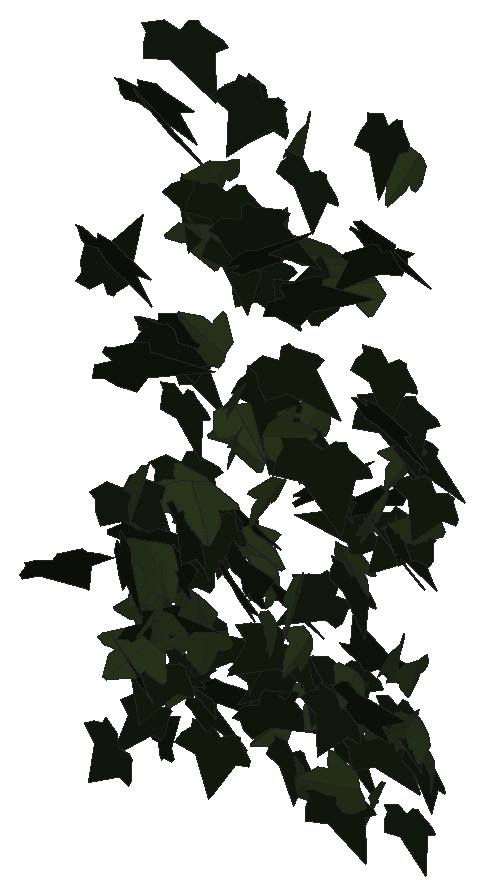
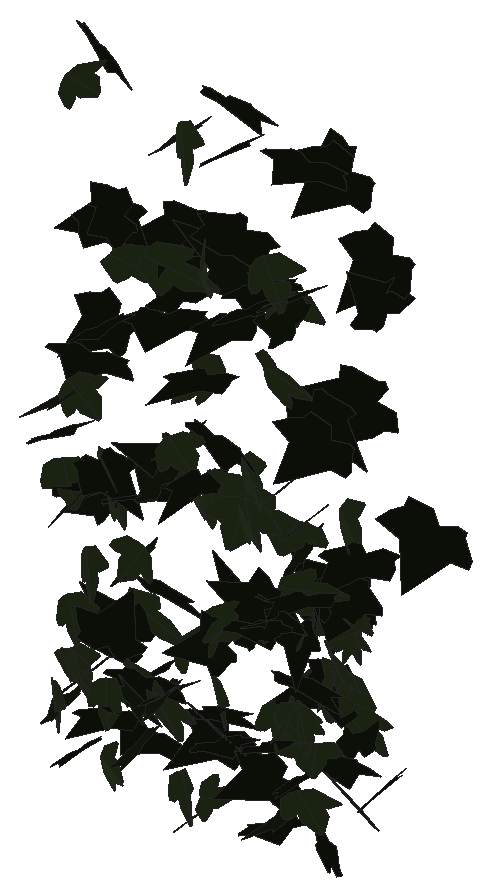
# SketchUp Ruby script. Lengths in inches.
U = 1.inch
M = Sketchup.active_model
def pt(a) = Geom::Point3d.new(a.map { |v| v * U })
def face(e, loops, mat)
  f = e.add_face(loops[0].map { |a| pt(a) })
  loops[1..].each { |l| e.add_face(l.map { |a| pt(a) }).erase! }
  f.material = f.back_material = mat if mat
  f
end
# faces: each face lists its corners as indices into pts; further lists are holes
def faces(e, pts, list, mat = nil) = list.each { |f| face(e, (f[0].is_a?(Array) ? f : [f]).map { |l| l.map { |i| pts[i] } }, mat) }
# xy, xz, yz: faces in a plane at the given z, y or x. An outline is a flat list of corners, or four numbers for a rectangle; further outlines are holes
def ring(l) = l.size == 4 ? [[l[0], l[1]], [l[2], l[1]], [l[2], l[3]], [l[0], l[3]]] : l.each_slice(2).to_a
def flat(e, list, mat, &to3) = list.each { |f| face(e, (f[0].is_a?(Array) ? f : [f]).map { |l| ring(l).map { |u, v| to3.(u, v) } }, mat) }
def xy(e, z, list, mat = nil) = flat(e, list, mat) { |x, y| [x, y, z] }
def xz(e, y, list, mat = nil) = flat(e, list, mat) { |x, z| [x, y, z] }
def yz(e, x, list, mat = nil) = flat(e, list, mat) { |y, z| [x, y, z] }
def lines(e, pts, list) = list.each { |a, b| e.add_line(pt(pts[a]), pt(pts[b])) }
# prism: a flat outline (further loops are holes) pulled along v
def prism(e, loops, v, mat = nil)
  f = face(e, loops, mat); d = Geom::Vector3d.new(v.map { |x| x * U })
  f.pushpull(f.normal.samedirection?(d) ? d.length : -d.length)
end
def box(e, o, s, mat = nil) = prism(e, [[o, [o[0] + s[0], o[1], o[2]], [o[0] + s[0], o[1] + s[1], o[2]], [o[0], o[1] + s[1], o[2]]]], [0, 0, s[2]], mat)
def at(x, y, z, deg = 0) = Geom::Transformation.translation(pt([x, y, z])) * Geom::Transformation.rotation(ORIGIN, Z_AXIS, deg.degrees)
def axes(o, x, y, z) = Geom::Transformation.new([*x, 0, *y, 0, *z, 0, *pt(o).to_a, 1])
def part(name) = M.definitions.add(name)
# library, detail: a bought-in or finely detailed component or shape, given as its bounding box
def library(name, o, s) = part(name).tap { |d| box(d.entities, o, s) }
def detail(e, o, s) = box(e.add_group.entities, o, s)
def put(e, d, t, mat = nil) = e.add_instance(d, t).tap { |i| i.material = mat if mat }
def group(e, t, mat = nil) = e.add_group.tap { |g| g.transformation = t; g.material = mat if mat }.entities
root = M.entities
M.materials.add("1026 AP 7946 SUNNY SIDE UP").color = [254, 231, 186]
M.materials.add("efeu1").color = [18, 25, 13]
M.materials.add("efeu2").color = [43, 57, 29]
c1 = part("ivyleaf_10")
p = [[0,0.5,-0.03],[-0.0625,2.02,-0.43],[-0.19,2.01,-0.46],[-0.54,1.05,-0.29],[-0.52,0.625,-0.18],[-0.83,0.76,-0.28],
  [-1.16,0.64,-0.33],[-1.15,0.33,-0.24],[-0.77,-0.39,0.02],[-0.3,-0.51,0.16],[0.04,-0.48,0.23],[-0.02,2.01,-0.4375],
  [-0.06,2.01,-0.43],[0.04,-0.49,0.23],[0.67,-0.49,0.14],[1.38,0.36,-0.2],[1.375,0.51,-0.24],[0.81,0.65,-0.19],
  [0.62,0.59,-0.15],[0.6,1.09,-0.28],[0.5,1.23,-0.31]]
faces(c1.entities,p,[[0,1,2,3,4,5,6,7,8,9,10],[11,12,0,13,14,15,16,17,18,19,20]],"efeu2")
c2 = part("ivyleaf_9")
p = [[1.54,2.16,1.25],[1.36,2.04,1.19],[-0.21,0.99,0.68],[-0.71,1.11,0.82],[-0.85,0.86,0.67],[-0.8,0.17,0.21],
  [-0.9,-0.01,0.1],[-0.67,-0.16,-0.02],[-0.08,-0.08,-0.05],[-0.03,-0.6,-0.4],[0.65,-0.88,-0.66],[0.83,-0.6,-0.49],
  [1.29,-0.42,-0.43],[1.8125,-0.07,-0.26],[1.21,0.44,0.15]]
faces(c2.entities,p,[[0,1,2,3,4,5,6,7,8,9,10,11,12,13,14]],"efeu1")
put(root,c1,axes([100.12,211.3,271],[0.10426,0.01974,-0.31622],[0.13596,0.28957,0.04256],[0.48425,-0.08555,0.05614]),"1026 AP 7946 SUNNY SIDE UP")
put(root,c2,axes([100.05,212,267.63],[-0.08362,0.11743,0.25344],[0.06935,-0.23297,0.13043],[0.44084,0.05892,0.02755]),"1026 AP 7946 SUNNY SIDE UP")
put(root,c1,axes([100.32,212.28,268.66],[-0.3053,-0.14792,0.11096],[-0.06583,-0.11387,-0.24313],[0.30139,-0.17471,0.0593]),"1026 AP 7946 SUNNY SIDE UP")
put(root,c1,axes([100.13,212.25,269.55],[0.30817,0.19972,-0.01399],[0.00499,-0.0238,-0.28862],[-0.34003,0.18065,-0.01692]),"1026 AP 7946 SUNNY SIDE UP")
put(root,c2,axes([100.04,212.0625,274.48],[0.44588,0.13162,0.0356],[0.0607,-0.00108,-0.31403],[-0.22159,0.26455,-0.01439]),"1026 AP 7946 SUNNY SIDE UP")
put(root,c1,axes([100.34,211.18,269.6],[0.48212,-0.03842,-0.13653],[-0.21895,-0.00921,-0.30586],[0.05308,0.31099,-0.02152]),"1026 AP 7946 SUNNY SIDE UP")
put(root,c2,axes([100.23,210.79,268.09],[-0.11983,-0.18972,0.23733],[-0.10766,-0.21525,-0.21943],[0.48675,-0.09431,0.00989]),"1026 AP 7946 SUNNY SIDE UP")
put(root,c1,axes([100.41,212.26,270.01],[-0.40465,0.08846,0.08291],[-0.14594,-0.01547,-0.26858],[-0.13426,-0.24981,0.04206]),"1026 AP 7946 SUNNY SIDE UP")
put(root,c2,axes([100.18,210.58,275.89],[-0.13022,-0.09744,0.34446],[0.41276,0.2137,0.13382],[-0.39708,0.25409,0.02613]),"1026 AP 7946 SUNNY SIDE UP")
put(root,c2,axes([100.42,212.29,270.58],[-0.43707,-0.07632,-0.02277],[0.04418,-0.01672,-0.28664],[0.12656,-0.25773,0.02141]),"1026 AP 7946 SUNNY SIDE UP")
put(root,c2,axes([100.24,209.35,271.8],[0.3327,0.28835,0.04603],[0.06901,0.01971,-0.37221],[-0.48915,0.1989,-0.02121]),"1026 AP 7946 SUNNY SIDE UP")
put(root,c2,axes([100.43,211.42,268.54],[-0.44747,0.07041,-0.12985],[0.18361,-0.06534,-0.29097],[-0.15367,-0.28311,0.03046]),"1026 AP 7946 SUNNY SIDE UP")
put(root,c2,axes([100.14,211.25,269.14],[-0.09609,-0.05725,0.30488],[0.10092,-0.28702,-0.053],[0.48393,0.04849,0.07159]),"1026 AP 7946 SUNNY SIDE UP")
put(root,c2,axes([100.33,211.69,269.07],[-0.37954,-0.16306,-0.07102],[0.11667,0.01415,-0.29451],[0.27366,-0.23219,0.02707]),"1026 AP 7946 SUNNY SIDE UP")
put(root,c2,axes([100.1,211.52,278.56],[0.54568,0.02421,-0.01707],[-0.02331,-0.03316,-0.34387],[-0.04368,0.32015,-0.02978]),"1026 AP 7946 SUNNY SIDE UP")
put(root,c2,axes([100.4,212.26,271.43],[0.30396,-0.00907,-0.23007],[-0.35023,0.016,-0.19924],[0.02835,0.2949,0.00547]),"1026 AP 7946 SUNNY SIDE UP")
put(root,c2,axes([100.16,211.09,272.17],[-0.02827,-0.18145,-0.27774],[0.04556,0.25567,-0.1915],[0.53219,-0.03152,0.00164]),"1026 AP 7946 SUNNY SIDE UP")
put(root,c2,axes([100.13,212.39,279.11],[-0.18262,-0.17835,-0.23486],[0.29834,0.1386,-0.21324],[0.37204,-0.19868,0.05571]),"1026 AP 7946 SUNNY SIDE UP")
put(root,c1,axes([100.35,212.08,271.36],[-0.11595,0.27724,-0.004],[-0.0542,-0.01538,-0.30363],[-0.46766,-0.06696,0.03618]),"1026 AP 7946 SUNNY SIDE UP")
put(root,c1,axes([100.61,212.11,271.88],[-0.05718,-0.00415,0.30413],[-0.22453,-0.26013,-0.02341],[0.40639,-0.1443,0.02986]),"1026 AP 7946 SUNNY SIDE UP")
put(root,c1,axes([100.43,211.31,270.14],[-0.53085,0.01348,-0.01798],[0.02648,-0.03033,-0.33402],[-0.02554,-0.31171,0.02732]),"1026 AP 7946 SUNNY SIDE UP")
put(root,c2,axes([100.19,212.36,272.04],[0.00898,-0.24206,-0.17505],[0.10532,0.16523,-0.24117],[0.45168,-0.03372,0.05972]),"1026 AP 7946 SUNNY SIDE UP")
put(root,c2,axes([100.25,212.29,273.2],[0.07098,-0.2812,0.01728],[-0.00153,-0.01875,-0.29348],[0.44309,0.04498,-0.00378]),"1026 AP 7946 SUNNY SIDE UP")
put(root,c2,axes([100.73,211.52,274.61],[0.12325,0.06216,-0.31135],[-0.44211,-0.13294,-0.1016],[-0.24648,0.26953,0.02656]),"1026 AP 7946 SUNNY SIDE UP")
put(root,c1,axes([100.58,211.31,270.07],[0.00582,0.02438,0.33164],[-0.23666,0.28478,-0.01878],[-0.44884,-0.14984,0.0142]),"1026 AP 7946 SUNNY SIDE UP")
put(root,c1,axes([100.46,211.33,270.45],[0.37061,-0.22088,0.03729],[0.02472,-0.03855,-0.33255],[0.37958,0.21817,-0.01475]),"1026 AP 7946 SUNNY SIDE UP")
put(root,c2,axes([100.3,210.34,276.625],[0.58653,-0.04429,-0.09819],[-0.15703,-0.00565,-0.37258],[0.07022,0.35729,-0.013]),"1026 AP 7946 SUNNY SIDE UP")
put(root,c1,axes([100.5,211.16,271],[0.42985,-0.18891,0.0138],[-0.00313,-0.02808,-0.33767],[0.32173,0.25212,-0.02172]),"1026 AP 7946 SUNNY SIDE UP")
put(root,c2,axes([100.36,212.27,273.93],[0.18364,-0.24619,-0.09937],[-0.04183,0.09245,-0.27976],[0.41285,0.11887,0.01586]),"1026 AP 7946 SUNNY SIDE UP")
put(root,c2,axes([100.56,211.125,271.58],[0.41527,0.15689,-0.15292],[-0.18311,-0.09936,-0.31156],[-0.31287,0.26639,-0.02063]),"1026 AP 7946 SUNNY SIDE UP")
put(root,c1,axes([100.52,211.02,272.59],[0.10492,-0.30171,0.12098],[0.09773,-0.1069,-0.32934],[0.54052,0.07789,0.03606]),"1026 AP 7946 SUNNY SIDE UP")
put(root,c2,axes([100.4,212.23,268.99],[0.0854,-0.24109,-0.08674],[-0.02812,0.0761,-0.26261],[0.42917,0.05296,0.00006]),"1026 AP 7946 SUNNY SIDE UP")
put(root,c2,axes([100.3125,210.81,271.37],[-0.01245,-0.03388,-0.35707],[0.53727,-0.10935,0.00292],[-0.18534,-0.31471,0.03245]),"1026 AP 7946 SUNNY SIDE UP")
put(root,c2,axes([100.26,210.76,274.48],[0.15346,0.15583,-0.306],[0.16511,0.27236,0.19435],[0.53056,-0.12983,0.02802]),"1026 AP 7946 SUNNY SIDE UP")
put(root,c2,axes([100.42,211.22,270.02],[0.01711,0.10881,-0.30875],[0.03847,0.28893,0.12101],[0.5241,-0.02476,0.0012]),"1026 AP 7946 SUNNY SIDE UP")
put(root,c1,axes([100.59,211.17,271.28],[-0.51625,-0.02427,-0.09955],[0.16258,-0.08379,-0.31416],[-0.00356,-0.30668,0.08909]),"1026 AP 7946 SUNNY SIDE UP")
put(root,c1,axes([100.42,212.33,269.82],[0.08139,-0.08172,0.28289],[0.39044,-0.12731,-0.08785],[0.22611,0.24925,0.04987]),"1026 AP 7946 SUNNY SIDE UP")
put(root,c1,axes([100.67,212.23,269.8],[-0.10908,0.26712,-0.01969],[-0.00026,-0.02253,-0.29438],[-0.45496,-0.06403,0.00489]),"1026 AP 7946 SUNNY SIDE UP")
put(root,c2,axes([100.67,212.26,276.625],[-0.16142,-0.26471,0.09657],[0.00392,-0.10224,-0.29056],[0.44233,-0.0957,0.03782]),"1026 AP 7946 SUNNY SIDE UP")
put(root,c1,axes([100.85,212.39,277.14],[-0.16678,-0.29205,0.05493],[-0.01187,-0.05571,-0.3202],[0.46714,-0.10569,0.01148]),"1026 AP 7946 SUNNY SIDE UP")
put(root,c2,axes([100.58,212.24,268.35],[0.27926,-0.16816,-0.1071],[-0.04631,0.10693,-0.24436],[0.32701,0.15875,0.05685]),"1026 AP 7946 SUNNY SIDE UP")
put(root,c2,axes([100.54,212.23,276.28],[0.22272,-0.23591,0.1124],[0.0981,-0.09133,-0.28394],[0.39766,0.15466,0.00709]),"1026 AP 7946 SUNNY SIDE UP")
put(root,c2,axes([100.47,211.33,278.4],[0.31506,-0.21696,0.16287],[0.16032,-0.12307,-0.30728],[0.42325,0.20812,-0.00485]),"1026 AP 7946 SUNNY SIDE UP")
put(root,c2,axes([100.9,212.46,269.42],[-0.27503,-0.18843,0.08124],[-0.0361,-0.08642,-0.26213],[0.31981,-0.1718,0.04028]),"1026 AP 7946 SUNNY SIDE UP")
put(root,c2,axes([100.75,212.33,271.58],[-0.3241,-0.06974,-0.21134],[0.32113,0.03039,-0.22229],[0.112,-0.28893,0.02582]),"1026 AP 7946 SUNNY SIDE UP")
put(root,c1,axes([101,211.875,269.68],[-0.27302,-0.24402,0.00536],[0.01905,-0.01668,-0.30797],[0.38336,-0.17296,0.01912]),"1026 AP 7946 SUNNY SIDE UP")
put(root,c1,axes([100.94,211.84,276.36],[-0.42321,-0.11538,-0.06051],[0.10182,-0.00436,-0.30022],[0.17575,-0.27531,0.02822]),"1026 AP 7946 SUNNY SIDE UP")
put(root,c2,axes([101.03,212.5,271.35],[-0.28516,-0.21246,-0.04147],[0.05982,0.01878,-0.28715],[0.33435,-0.18456,0.016]),"1026 AP 7946 SUNNY SIDE UP")
put(root,c2,axes([101.05,212.11,267.94],[-0.19315,-0.25656,-0.01156],[0.01776,0.00541,-0.29289],[0.40331,-0.12311,0.00736]),"1026 AP 7946 SUNNY SIDE UP")
put(root,c2,axes([100.86,211.3,271.09],[0.00241,-0.00856,0.33625],[0.13703,-0.3146,-0.01076],[0.49485,0.08716,0.00134]),"1026 AP 7946 SUNNY SIDE UP")
put(root,c2,axes([100.99,212.35,276.77],[-0.1061,-0.29336,-0.0957],[0.06675,0.0836,-0.30882],[0.47844,-0.07672,0.02187]),"1026 AP 7946 SUNNY SIDE UP")
put(root,c2,axes([101.05,212.03,271.62],[-0.14489,-0.28388,0.00778],[0.00497,-0.01066,-0.30747],[0.44659,-0.09198,0.00595]),"1026 AP 7946 SUNNY SIDE UP")
put(root,c1,axes([101.5,211.52,274.82],[0.12878,0.05298,0.32897],[-0.4975,0.08122,0.07026],[-0.10521,-0.3192,0.07044]),"1026 AP 7946 SUNNY SIDE UP")
put(root,c2,axes([100.91,212.09,268.73],[0.4062,0.06017,0.0958],[0.15222,0.0065,-0.26359],[-0.09967,0.25511,-0.01212]),"1026 AP 7946 SUNNY SIDE UP")
put(root,c1,axes([101.29,212.29,273.7],[0.08514,-0.28283,0.00567],[-0.00417,-0.00775,-0.29667],[0.44484,0.05406,-0.00386]),"1026 AP 7946 SUNNY SIDE UP")
put(root,c1,axes([101.28,212.36,272.98],[0.11351,-0.26584,0.07438],[0.02916,-0.07135,-0.2842],[0.4328,0.07453,-0.00036]),"1026 AP 7946 SUNNY SIDE UP")
put(root,c2,axes([100.95,212.41,271.62],[0.22584,-0.15305,0.21347],[0.22133,-0.15326,-0.21712],[0.34057,0.2011,-0.00046]),"1026 AP 7946 SUNNY SIDE UP")
put(root,c2,axes([101.18,211.28,271.81],[-0.01941,-0.18489,0.28044],[-0.02284,-0.27289,-0.19248],[0.5183,-0.01895,0.00202]),"1026 AP 7946 SUNNY SIDE UP")
put(root,c1,axes([101.38,212.3125,273],[-0.44392,-0.10538,-0.05405],[0.08841,-0.00271,-0.30964],[0.16214,-0.28703,0.02086]),"1026 AP 7946 SUNNY SIDE UP")
put(root,c1,axes([101.21,211.34,272.38],[0.45962,0.11822,0.10393],[0.16422,0.0078,-0.32326],[-0.18004,0.30891,-0.02954]),"1026 AP 7946 SUNNY SIDE UP")
put(root,c2,axes([101.41,212.15,276.17],[-0.07977,-0.30642,-0.03308],[0.01296,0.02942,-0.31978],[0.48401,-0.05129,0.00311]),"1026 AP 7946 SUNNY SIDE UP")
put(root,c1,axes([101.38,212.29,271.29],[-0.27434,-0.15177,-0.19831],[0.28021,0.0822,-0.23373],[0.26312,-0.24578,0.04215]),"1026 AP 7946 SUNNY SIDE UP")
put(root,c1,axes([101.34,212.21,273.3125],[0.38461,0.09351,0.16058],[0.23948,0.03558,-0.26891],[-0.1547,0.28757,-0.01706]),"1026 AP 7946 SUNNY SIDE UP")
put(root,c2,axes([101.89,212.47,269.64],[-0.36472,-0.11204,0.0738],[-0.07445,-0.06636,-0.2629],[0.19598,-0.23371,0.03747]),"1026 AP 7946 SUNNY SIDE UP")
put(root,c2,axes([101.74,212.44,269.17],[-0.1985,-0.23294,0.01366],[0.00523,-0.01837,-0.27279],[0.36696,-0.12574,0.01128]),"1026 AP 7946 SUNNY SIDE UP")
put(root,c1,axes([101.86,212.54,268.29],[0.01337,0.08367,-0.2621],[-0.15823,-0.23541,-0.08445],[-0.39104,0.09812,0.02521]),"1026 AP 7946 SUNNY SIDE UP")
put(root,c2,axes([101.54,211.82,270.76],[0.05063,-0.12832,0.28256],[0.14792,-0.2587,-0.13722],[0.45367,0.09867,0.01321]),"1026 AP 7946 SUNNY SIDE UP")
put(root,c1,axes([101.85,212.3,269.98],[0.22979,-0.20748,-0.10849],[-0.0488,0.10448,-0.25872],[0.36176,0.14589,0.03401]),"1026 AP 7946 SUNNY SIDE UP")
put(root,c2,axes([101.79,212.27,278.61],[-0.1821,-0.23925,0.16185],[-0.05061,-0.15898,-0.27243],[0.44839,-0.11511,0.03498]),"1026 AP 7946 SUNNY SIDE UP")
put(root,c1,axes([101.79,212.35,270.76],[-0.15123,-0.01602,0.28643],[0.13946,-0.28069,0.01329],[0.41526,0.08843,0.09985]),"1026 AP 7946 SUNNY SIDE UP")
put(root,c2,axes([101.74,212.16,275.85],[0.01879,-0.20786,-0.24076],[-0.01046,0.23247,-0.21308],[0.4903,0.01293,0.00468]),"1026 AP 7946 SUNNY SIDE UP")
put(root,c2,axes([101.91,212.27,273.98],[-0.37688,-0.05829,-0.19493],[0.29681,0.02065,-0.25321],[0.09228,-0.30447,0.01829]),"1026 AP 7946 SUNNY SIDE UP")
put(root,c2,axes([102.15,212.26,269.375],[-0.39121,0.07735,-0.059],[0.06688,-0.05536,-0.26567],[-0.13621,-0.24933,0.03902]),"1026 AP 7946 SUNNY SIDE UP")
put(root,c2,axes([101.74,211.8,270.98],[-0.01716,-0.0028,0.31286],[0.19672,-0.27697,0.00038],[0.43517,0.12509,0.01217]),"1026 AP 7946 SUNNY SIDE UP")
put(root,c2,axes([101.71,212.3125,270.7],[0.39876,-0.13952,0.08994],[0.10206,-0.06417,-0.29754],[0.23854,0.26068,-0.02305]),"1026 AP 7946 SUNNY SIDE UP")
put(root,c2,axes([102.2,211.62,279.07],[-0.44386,-0.08578,-0.10064],[0.1645,-0.01318,-0.30108],[0.12039,-0.29826,0.04036]),"1026 AP 7946 SUNNY SIDE UP")
put(root,c2,axes([102.08,212.5,267.89],[-0.00698,-0.24455,0.08008],[-0.00728,-0.07904,-0.25242],[0.40409,-0.00565,-0.00316]),"1026 AP 7946 SUNNY SIDE UP")
put(root,c2,axes([102.05,211.86,268.96],[-0.00924,-0.01387,-0.31412],[0.00725,0.30486,-0.0126],[0.47977,-0.00487,-0.00586]),"1026 AP 7946 SUNNY SIDE UP")
put(root,c2,axes([101.97,211.54,276.34],[0.20187,0.30471,-0.05223],[0.00894,0.05444,0.34057],[0.48609,-0.12754,0.01543]),"1026 AP 7946 SUNNY SIDE UP")
put(root,c2,axes([101.95,211.58,277],[0.02492,-0.0632,-0.33849],[0.17861,0.31005,-0.05404],[0.49429,-0.10885,0.03659]),"1026 AP 7946 SUNNY SIDE UP")
put(root,c1,axes([102.04,212.37,276.625],[0.08456,-0.05904,0.30729],[0.29364,-0.23307,-0.08348],[0.37798,0.19427,-0.00389]),"1026 AP 7946 SUNNY SIDE UP")
put(root,c1,axes([102.31,211.8,272.67],[-0.00122,-0.27479,0.15408],[0.00647,-0.15112,-0.28394],[0.49307,0.0013,0.00411]),"1026 AP 7946 SUNNY SIDE UP")
put(root,c2,axes([102.1875,212.27,273.23],[0.06269,-0.20331,-0.23824],[-0.07139,0.22559,-0.21212],[0.47751,0.06042,-0.00043]),"1026 AP 7946 SUNNY SIDE UP")
put(root,c1,axes([102.54,212.4,273.67],[-0.18971,-0.22652,0.154],[0.03151,-0.17188,-0.25051],[0.42671,-0.08802,0.08697]),"1026 AP 7946 SUNNY SIDE UP")
put(root,c1,axes([102.92,212.27,276.46],[0.11573,0.08704,-0.30885],[-0.49115,0.03379,-0.06858],[0.02122,0.30732,0.09697]),"1026 AP 7946 SUNNY SIDE UP")
put(root,c1,axes([102.62,212.08,278.54],[0.04868,-0.30686,-0.10182],[0.01449,0.09834,-0.31661],[0.50588,0.02671,0.01887]),"1026 AP 7946 SUNNY SIDE UP")
put(root,c2,axes([102.35,211.94,274.67],[0.07808,-0.20146,-0.24288],[0.0933,0.23942,-0.19745],[0.47723,-0.01384,0.07834]),"1026 AP 7946 SUNNY SIDE UP")
put(root,c1,axes([102.81,211.92,267.93],[-0.25752,0.12108,0.19592],[-0.26446,0.08964,-0.20824],[-0.23469,-0.23387,0.01968]),"1026 AP 7946 SUNNY SIDE UP")
put(root,c1,axes([102.69,211.99,270.16],[-0.06452,-0.11633,0.27846],[0.1352,-0.2664,-0.10597],[0.44352,0.06429,0.07281]),"1026 AP 7946 SUNNY SIDE UP")
put(root,c2,axes([102.81,211.88,275.73],[-0.22732,-0.0937,0.2761],[0.33983,0.15963,0.17818],[-0.29072,0.25987,-0.00761]),"1026 AP 7946 SUNNY SIDE UP")
put(root,c2,axes([102.6875,212.11,273.56],[0.02532,-0.28087,0.07037],[0.02274,-0.06914,-0.29004],[0.45455,0.01911,0.01059]),"1026 AP 7946 SUNNY SIDE UP")
put(root,c2,axes([102.7,212.43,269.55],[0.17361,-0.24542,0.00284],[-0.01088,-0.00767,-0.27711],[0.3858,0.11022,-0.0091]),"1026 AP 7946 SUNNY SIDE UP")
put(root,c2,axes([102.84,212.3,269.5],[-0.13108,-0.24478,0.08584],[-0.00331,-0.08835,-0.26564],[0.40728,-0.0795,0.02547]),"1026 AP 7946 SUNNY SIDE UP")
put(root,c1,axes([102.93,212.22,269.3125],[0.4653,-0.0701,-0.03678],[-0.06327,-0.01726,-0.31225],[0.10596,0.29752,-0.02494]),"1026 AP 7946 SUNNY SIDE UP")
put(root,c2,axes([103.16,212.07,271.06],[-0.43265,0.00776,0.01551],[-0.02454,-0.023,-0.28268],[-0.01017,-0.2746,0.0225]),"1026 AP 7946 SUNNY SIDE UP")
put(root,c1,axes([102.68,212.14,273.16],[0.21791,-0.05687,0.28091],[0.38179,-0.12532,-0.15461],[0.21564,0.27934,-0.01014]),"1026 AP 7946 SUNNY SIDE UP")
put(root,c1,axes([102.98,211.02,274.0625],[0.0172,0.07602,0.35227],[-0.03674,0.34108,-0.07545],[-0.54891,-0.02045,0.01609]),"1026 AP 7946 SUNNY SIDE UP")
put(root,c2,axes([102.85,212.3125,272.92],[0.10769,-0.24382,0.17277],[0.10843,-0.15571,-0.26098],[0.45378,0.09507,0.02136]),"1026 AP 7946 SUNNY SIDE UP")
put(root,c2,axes([102.97,211.72,272.83],[0.06404,0.29298,-0.12331],[-0.00635,0.12283,0.3048],[0.49861,-0.03607,0.01972]),"1026 AP 7946 SUNNY SIDE UP")
put(root,c2,axes([103.07,211.67,278.14],[-0.03701,-0.29082,0.10136],[0.0284,-0.10146,-0.30009],[0.48275,-0.01633,0.02543]),"1026 AP 7946 SUNNY SIDE UP")
put(root,c2,axes([103.1,212.36,269.69],[-0.23294,-0.1758,-0.1905],[0.2311,0.11459,-0.23413],[0.32656,-0.2065,0.0298]),"1026 AP 7946 SUNNY SIDE UP")
put(root,c2,axes([103.36,212.46,269.49],[-0.29309,0.09621,-0.17194],[0.19145,-0.12209,-0.21261],[-0.2357,-0.2188,0.0411]),"1026 AP 7946 SUNNY SIDE UP")
put(root,c1,axes([103.58,212.25,276.27],[0.23834,0.03591,-0.27418],[-0.3987,-0.08228,-0.16056],[-0.14012,0.29521,-0.00951]),"1026 AP 7946 SUNNY SIDE UP")
put(root,c1,axes([103.35,212.22,269.67],[0.40981,-0.16523,-0.02872],[-0.05735,-0.00739,-0.31685],[0.25692,0.26191,-0.02492]),"1026 AP 7946 SUNNY SIDE UP")
put(root,c1,axes([103.27,212.34,271.65],[-0.36837,0.12655,-0.07986],[0.09614,-0.05115,-0.27415],[-0.21327,-0.24164,0.01434]),"1026 AP 7946 SUNNY SIDE UP")
put(root,c2,axes([103.12,211.14,276.37],[0.06145,0.16111,-0.31845],[0.05405,0.30867,0.17152],[0.54672,-0.04862,0.01883]),"1026 AP 7946 SUNNY SIDE UP")
put(root,c2,axes([103.16,212.39,268.59],[0.2036,-0.26098,-0.03446],[-0.04201,0.02239,-0.29966],[0.4113,0.13148,-0.01355]),"1026 AP 7946 SUNNY SIDE UP")
put(root,c2,axes([103.72,212.22,272.27],[-0.28473,0.04112,0.21695],[-0.3042,-0.14991,-0.14225],[0.14509,-0.2336,0.12751]),"1026 AP 7946 SUNNY SIDE UP")
put(root,c2,axes([103.46,211.85,269.4],[-0.13474,-0.24762,0.14405],[-0.04357,-0.13955,-0.27018],[0.44612,-0.08842,0.01712]),"1026 AP 7946 SUNNY SIDE UP")
put(root,c2,axes([103.4,212.22,271.36],[0.06836,-0.27556,0.11619],[0.01756,-0.11397,-0.28798],[0.46878,0.04446,-0.00615]),"1026 AP 7946 SUNNY SIDE UP")
put(root,c1,axes([103.59,210.72,271.97],[0.24585,-0.22714,0.22593],[0.18653,-0.18609,-0.2851],[0.46161,0.19617,-0.00512]),"1026 AP 7946 SUNNY SIDE UP")
put(root,c1,axes([103.74,212.28,272.4375],[0.08959,-0.26689,0.06797],[0.04264,-0.06315,-0.2812],[0.43076,0.06176,0.01369]),"1026 AP 7946 SUNNY SIDE UP")
put(root,c2,axes([103.79,212.33,270.01],[0.33691,-0.10423,0.18616],[-0.22461,0.11662,0.24368],[-0.24015,-0.2553,0.03325]),"1026 AP 7946 SUNNY SIDE UP")
put(root,c2,axes([103.9,212.35,272.89],[-0.05172,0.20859,-0.19439],[-0.01202,-0.19175,-0.21677],[-0.44336,-0.01914,0.02856]),"1026 AP 7946 SUNNY SIDE UP")
put(root,c2,axes([103.9375,212.21,276.89],[-0.01032,0.18177,-0.25764],[-0.03189,-0.25089,-0.188],[-0.4864,0.01259,0.0178]),"1026 AP 7946 SUNNY SIDE UP")
put(root,c1,axes([103.875,212.25,269.2],[-0.14843,-0.254,-0.04442],[0.02426,0.03873,-0.27893],[0.404,-0.09565,0.00043]),"1026 AP 7946 SUNNY SIDE UP")
put(root,c2,axes([103.55,212.34,277.03],[0.43497,-0.09137,0.08882],[0.11542,-0.05319,-0.29921],[0.161,0.28499,-0.02547]),"1026 AP 7946 SUNNY SIDE UP")
put(root,c1,axes([103.86,212.26,268.02],[0.13027,-0.20521,0.15771],[0.08516,-0.14447,-0.22881],[0.39459,0.09893,-0.00269]),"1026 AP 7946 SUNNY SIDE UP")
put(root,c1,axes([103.92,212.25,272.83],[0.23113,-0.24032,0.0265],[0.003,-0.03054,-0.29002],[0.38026,0.14631,-0.01382]),"1026 AP 7946 SUNNY SIDE UP")
put(root,c2,axes([103.75,211.45,268.19],[-0.19362,-0.11877,-0.23661],[0.31448,0.11632,-0.17226],[0.2562,-0.23254,0.03263]),"1026 AP 7946 SUNNY SIDE UP")
put(root,c2,axes([103.79,212.25,268.83],[0.00762,-0.18182,-0.21025],[0.11591,0.19639,-0.1782],[0.4126,-0.05181,0.05395]),"1026 AP 7946 SUNNY SIDE UP")
put(root,c2,axes([104,212.3,275.04],[-0.08047,-0.28909,0.03023],[-0.00067,-0.03139,-0.30259],[0.45717,-0.05093,0.00488]),"1026 AP 7946 SUNNY SIDE UP")
put(root,c2,axes([103.89,212.2,272.32],[0.35041,-0.16959,0.0236],[0.01245,-0.02893,-0.28806],[0.26901,0.22225,-0.01741]),"1026 AP 7946 SUNNY SIDE UP")
put(root,c2,axes([104.36,212.4,272.37],[-0.33162,-0.1742,0.07014],[-0.06005,-0.06186,-0.28119],[0.28847,-0.21313,0.0221]),"1026 AP 7946 SUNNY SIDE UP")
put(root,c2,axes([103.88,211.62,269.74],[0.39453,-0.03779,-0.20288],[0.31498,0.04565,0.25444],[-0.00169,-0.31555,0.0592]),"1026 AP 7946 SUNNY SIDE UP")
put(root,c2,axes([104.14,212.37,269.41],[0.0971,-0.27722,-0.00695],[-0.00134,0.00511,-0.29256],[0.43598,0.06176,0.00065]),"1026 AP 7946 SUNNY SIDE UP")
put(root,c2,axes([104.18,210.57,274.41],[-0.19538,-0.30123,-0.16762],[0.12451,0.14124,-0.33439],[0.52243,-0.14632,0.01701]),"1026 AP 7946 SUNNY SIDE UP")
put(root,c2,axes([104.22,212.28,272.41],[0.25411,-0.22051,-0.14488],[-0.1342,0.11024,-0.28097],[0.38761,0.18273,-0.0023]),"1026 AP 7946 SUNNY SIDE UP")
put(root,c2,axes([104.22,212.1875,274.48],[-0.22536,-0.19319,-0.20996],[0.24895,0.13192,-0.24407],[0.36318,-0.21031,0.03702]),"1026 AP 7946 SUNNY SIDE UP")
put(root,c1,axes([104.5,212.19,273.82],[-0.11901,-0.23413,0.16329],[-0.01694,-0.16294,-0.25209],[0.44543,-0.06875,0.03404]),"1026 AP 7946 SUNNY SIDE UP")
put(root,c1,axes([104.49,212.17,269.45],[-0.00515,-0.26824,0.02679],[-0.00034,-0.02753,-0.27652],[0.42399,-0.00328,0.0001]),"1026 AP 7946 SUNNY SIDE UP")
put(root,c1,axes([104.55,212.36,272.58],[-0.27342,-0.21855,0.04725],[-0.02863,-0.04564,-0.28763],[0.35038,-0.17428,0.01337]),"1026 AP 7946 SUNNY SIDE UP")
put(root,c2,axes([104.37,211.8125,279.27],[-0.33147,-0.02455,-0.26597],[0.40487,-0.05804,-0.21135],[-0.04682,-0.3281,0.0553]),"1026 AP 7946 SUNNY SIDE UP")
put(root,c1,axes([104.89,210.3,269.3],[-0.15994,0.04282,0.3322],[-0.51094,-0.02249,-0.10272],[0.01376,-0.33715,0.04703]),"1026 AP 7946 SUNNY SIDE UP")
put(root,c1,axes([104.54,212.22,270.32],[-0.0845,-0.27376,-0.02286],[0.01158,0.01958,-0.28727],[0.43153,-0.05413,0.00323]),"1026 AP 7946 SUNNY SIDE UP")
put(root,c1,axes([104.71,212.1,269.32],[0.22568,-0.11664,-0.2037],[-0.25189,0.11506,-0.18968],[0.25731,0.21494,-0.00702]),"1026 AP 7946 SUNNY SIDE UP")
put(root,c2,axes([104.3,211.56,274.74],[0.50279,-0.07206,-0.01786],[-0.03644,-0.02615,-0.33636],[0.11054,0.31914,-0.02962]),"1026 AP 7946 SUNNY SIDE UP")
put(root,c1,axes([104.61,211.74,270.82],[0.0438,-0.29439,-0.08364],[0.01973,0.08089,-0.30351],[0.47909,0.02359,0.02014]),"1026 AP 7946 SUNNY SIDE UP")
put(root,c1,axes([104.64,212.03,278.7],[-0.13548,-0.1908,0.25968],[0.09198,-0.26741,-0.18868],[0.48991,-0.00256,0.10724]),"1026 AP 7946 SUNNY SIDE UP")
put(root,c2,axes([104.45,212.31,273.85],[0.25157,-0.21575,-0.11107],[-0.00407,0.12645,-0.26693],[0.37836,0.14481,0.07098]),"1026 AP 7946 SUNNY SIDE UP")
put(root,c2,axes([104.54,212.08,267.91],[0.04134,-0.26016,-0.02744],[0.00146,0.02538,-0.26921],[0.41099,0.02608,0.00372]),"1026 AP 7946 SUNNY SIDE UP")
put(root,c2,axes([104.73,212.43,273.13],[-0.18829,-0.23747,0.09564],[-0.01154,-0.10078,-0.27197],[0.40154,-0.11425,0.03704]),"1026 AP 7946 SUNNY SIDE UP")
put(root,c2,axes([104.625,212.34,268.68],[0.02945,-0.23301,0.1321],[0.02784,-0.1285,-0.24148],[0.41828,0.02496,0.00677]),"1026 AP 7946 SUNNY SIDE UP")
put(root,c1,axes([104.85,212.2,268.82],[0.21853,-0.20139,-0.11293],[-0.0189,0.12032,-0.24529],[0.35918,0.12886,0.0558]),"1026 AP 7946 SUNNY SIDE UP")
